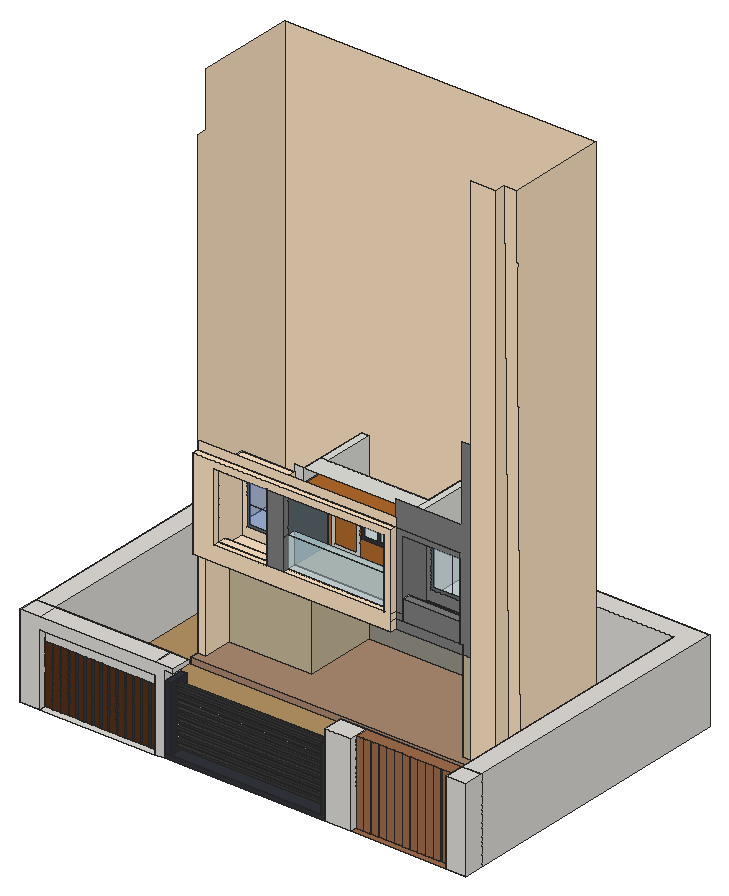
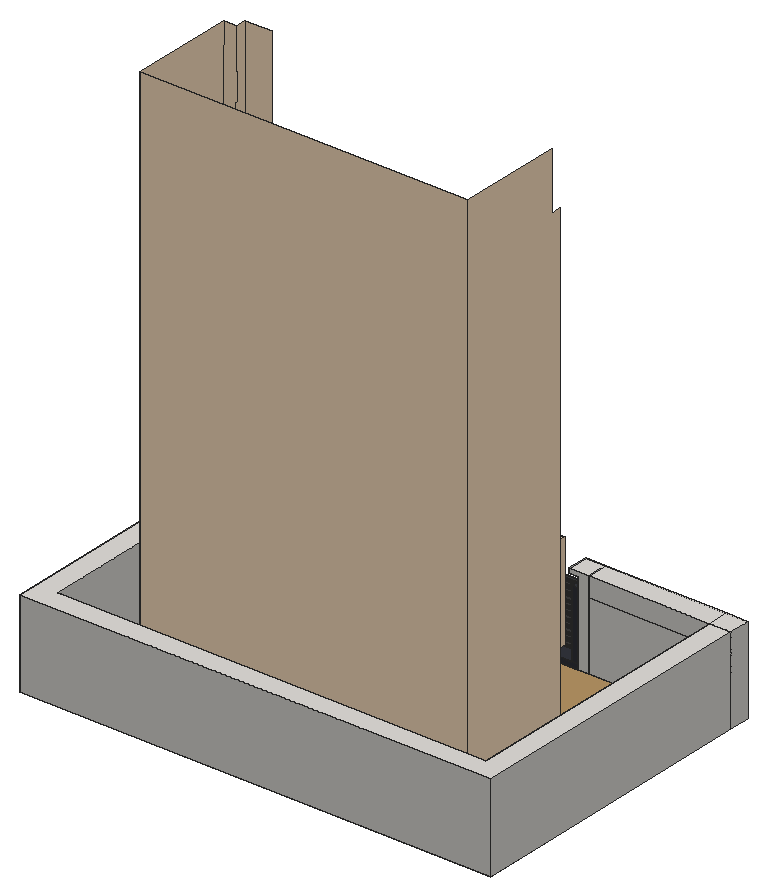
# SketchUp Ruby script. Lengths in inches.
U = 1.inch
M = Sketchup.active_model
def pt(a) = Geom::Point3d.new(a.map { |v| v * U })
def face(e, loops, mat)
  f = e.add_face(loops[0].map { |a| pt(a) })
  loops[1..].each { |l| e.add_face(l.map { |a| pt(a) }).erase! }
  f.material = f.back_material = mat if mat
  f
end
# faces: each face lists its corners as indices into pts; further lists are holes
def faces(e, pts, list, mat = nil) = list.each { |f| face(e, (f[0].is_a?(Array) ? f : [f]).map { |l| l.map { |i| pts[i] } }, mat) }
# xy, xz, yz: faces in a plane at the given z, y or x. An outline is a flat list of corners, or four numbers for a rectangle; further outlines are holes
def ring(l) = l.size == 4 ? [[l[0], l[1]], [l[2], l[1]], [l[2], l[3]], [l[0], l[3]]] : l.each_slice(2).to_a
def flat(e, list, mat, &to3) = list.each { |f| face(e, (f[0].is_a?(Array) ? f : [f]).map { |l| ring(l).map { |u, v| to3.(u, v) } }, mat) }
def xy(e, z, list, mat = nil) = flat(e, list, mat) { |x, y| [x, y, z] }
def xz(e, y, list, mat = nil) = flat(e, list, mat) { |x, z| [x, y, z] }
def yz(e, x, list, mat = nil) = flat(e, list, mat) { |y, z| [x, y, z] }
def lines(e, pts, list) = list.each { |a, b| e.add_line(pt(pts[a]), pt(pts[b])) }
# prism: a flat outline (further loops are holes) pulled along v
def prism(e, loops, v, mat = nil)
  f = face(e, loops, mat); d = Geom::Vector3d.new(v.map { |x| x * U })
  f.pushpull(f.normal.samedirection?(d) ? d.length : -d.length)
end
def box(e, o, s, mat = nil) = prism(e, [[o, [o[0] + s[0], o[1], o[2]], [o[0] + s[0], o[1] + s[1], o[2]], [o[0], o[1] + s[1], o[2]]]], [0, 0, s[2]], mat)
def at(x, y, z, deg = 0) = Geom::Transformation.translation(pt([x, y, z])) * Geom::Transformation.rotation(ORIGIN, Z_AXIS, deg.degrees)
def axes(o, x, y, z) = Geom::Transformation.new([*x, 0, *y, 0, *z, 0, *pt(o).to_a, 1])
def part(name) = M.definitions.add(name)
# library, detail: a bought-in or finely detailed component or shape, given as its bounding box
def library(name, o, s) = part(name).tap { |d| box(d.entities, o, s) }
def detail(e, o, s) = box(e.add_group.entities, o, s)
def put(e, d, t, mat = nil) = e.add_instance(d, t).tap { |i| i.material = mat if mat }
def group(e, t, mat = nil) = e.add_group.tap { |g| g.transformation = t; g.material = mat if mat }.entities
root = M.entities
M.materials.add("[0012_Bisque]").color = [255, 228, 196]
M.materials.add("[Carpet Pattern Leaf Squares Tan]").color = [181, 154, 125]
M.materials.add("[Color M07]").color = [58, 58, 58]
M.materials.add("[Formica Graystone]").color = [149, 146, 135]
M.materials.add("[Formica Laminate Dark]").color = [50, 53, 60]
M.materials.add("[Formica Speckled Grey]").color = [94, 105, 111]
M.materials.add("[Groundcover Sand Smooth]").color = [182, 148, 101]
M.materials.add("[Quartz Light Brown]").color = [199, 184, 152]
M.materials.add("[Slate Light Tile]").color = [127, 127, 127]
M.materials.add("[Terrazzo Tile Accent]").color = [224, 221, 217]
M.materials.add("[Terrazzo Tile Light]").color = [219, 217, 210]
M.materials.add("[Tile Veriegated Stone]").color = [171, 137, 112]
M.materials.add("[Translucent Glass Blue]").color = [100, 149, 237]
M.materials["[Translucent Glass Blue]"].alpha = 0.5
M.materials.add("[Translucent Glass Safety]").color = [204, 235, 244]
M.materials["[Translucent Glass Safety]"].alpha = 0.5
M.materials.add("[Wood Bamboo]").color = [177, 105, 43]
M.materials.add("[Wood Veneer 01]").color = [84, 49, 25]
M.materials.add("[Wood Veneer 02]").color = [160, 108, 76]
xy(root,0,[[0,0,26.06,26.06],[177.43,0,190.63,26.06],[190.63,0,401.35,26.06],[401.35,0,436.18,26.06],[561.76,0,587.8125,26.06],
  [26.06,8.35,177.43,26.06],[436.18,8.57,561.76,26.06],[0,26.06,0,401.5,587.8125,401.5,587.8125,26.06,561.76,26.06,561.76,375.44,26.06,375.44,26.06,26.06],[88.29,171.61,448.4,325.8],[448.4,171.61,498.52,325.8]])
xy(root,0,[[[26.06,26.06,561.76,375.44],[448.4,171.61,498.52,325.8]]],"[Groundcover Sand Smooth]")
xy(root,0,[[26.06,0,177.43,8.35]],"[Terrazzo Tile Accent]")
xy(root,0,[[436.18,0,561.76,8.57]],"[Wood Veneer 02]")
xy(root,6.0625,[[190.63,0,198.32,26.06],[396.54,0,401.35,26.06]])
xy(root,6.0625,[[198.32,0,396.54,26.06]],"[Formica Laminate Dark]")
xy(root,9,[[88.29,171.61,498.52,171.61,498.52,202.27,482.08,202.27,482.08,181.99,438.01,181.99,438.01,315.42,207.7,315.42,207.7,220.49,98.67,220.49,98.67,181.99,88.29,181.99]],"[Tile Veriegated Stone]")
xy(root,12.03,[[198.32,9.24,396.54,13.93]],"[Color M07]")
xy(root,15.03,[[198.32,9.24,396.54,13.93]],"[Color M07]")
xy(root,19.66,[[198.32,9.24,401.35,13.93]],"[Color M07]")
xy(root,22.66,[[198.32,9.24,401.35,13.93]],"[Color M07]")
xy(root,27.1,[[198.32,9.24,396.54,13.93]],"[Color M07]")
xy(root,30.1,[[198.32,9.24,396.54,13.93]],"[Color M07]")
xy(root,33.97,[[198.32,9.24,396.54,13.93]],"[Color M07]")
xy(root,36.97,[[198.32,9.24,396.54,13.93]],"[Color M07]")
xy(root,41.35,[[198.32,9.24,396.54,13.93]],"[Color M07]")
xy(root,44.35,[[198.32,9.24,396.54,13.93]],"[Color M07]")
xy(root,48.91,[[198.32,9.24,396.54,13.93]],"[Color M07]")
xy(root,51.91,[[198.32,9.24,396.54,13.93]],"[Color M07]")
xy(root,55.78,[[198.32,9.24,396.54,13.93]],"[Color M07]")
xy(root,58.78,[[198.32,9.24,396.54,13.93]],"[Color M07]")
xy(root,62.91,[[198.32,9.24,396.54,13.93]],"[Color M07]")
xy(root,65.91,[[198.32,9.24,396.54,13.93]],"[Color M07]")
xy(root,71.22,[[198.32,9.24,396.54,13.93]],"[Color M07]")
xy(root,74.22,[[198.32,9.24,396.54,13.93]],"[Color M07]")
xy(root,78.85,[[198.32,9.24,396.54,13.93]],"[Color M07]")
xy(root,81.85,[[198.32,9.24,396.54,13.93]],"[Color M07]")
xy(root,85.66,[[198.32,9.24,396.54,13.93]],"[Color M07]")
xy(root,88.66,[[198.32,9.24,396.54,13.93]],"[Color M07]")
xy(root,91.76,[[190.63,0,198.32,26.06],[396.54,0,401.35,26.06]],"[Formica Laminate Dark]")
xy(root,93.4375,[[26.06,0,177.43,8.35]])
xy(root,104.12,[[190.63,0,201.76,26.06]])
xy(root,109.3125,[[0,0,26.06,26.06],[26.06,0,177.43,26.06],[177.43,0,201.76,26.06],[401.35,0,436.18,26.06],[561.76,0,587.8125,26.06],
  [0,26.06,26.06,26.06,26.06,375.44,561.76,375.44,561.76,26.06,587.8125,26.06,587.8125,401.5,0,401.5]],"[Terrazzo Tile Accent]")
xy(root,109.3125,[[436.18,8.57,561.76,26.06]],"[Wood Veneer 02]")
xy(root,129,[[88.29,174.18,98.67,181.99],[98.67,174.18,207.7,181.99],[98.67,181.99,207.7,220.49],[98.67,220.49,207.7,315.42]])
xy(root,129,[[207.7,174.18,349.51,181.99],[207.7,181.99,438.01,315.42]],"[0012_Bisque]")
xy(root,141,[[358.38,181.99,434.83,192.87],[434.83,181.99,438.01,192.87],[98.67,192.87,116.04,220.49],[349.51,192.87,358.38,220.49],[434.83,192.87,438.01,220.49],
  [98.67,220.49,197.7,315.42],[349.51,220.49,438.01,315.42],[207.7,247.93,340.25,315.42]])
xy(root,141,[[116.04,192.87,186.07,220.49]],"[0012_Bisque]")
xy(root,149.5,[[186.07,174.18,207.7,181.99],[340.25,174.18,349.51,181.99],[207.7,181.99,340.25,192.87]])
xy(root,149.5,[[116.04,174.18,186.07,181.99],[207.7,174.18,340.25,181.99],[116.04,181.99,186.07,192.87]],"[0012_Bisque]")
xy(root,149.5,[[207.7,192.87,340.25,247.93]],"[Carpet Pattern Leaf Squares Tan]")
xy(root,149.5,[[358.38,192.87,434.83,220.49]],"[Formica Speckled Grey]")
xy(root,167,[[358.38,181.99,434.83,192.87]],"[Slate Light Tile]")
xy(root,189.8125,[[207.7,181.99,340.25,192.87]],"[Translucent Glass Safety]")
xy(root,239.83,[[220.34,200.24,219.16,200.39,218.06,200.85,217.11,201.58,216.39,202.52,215.93,203.62,215.78,204.8,215.93,205.98,216.39,207.08,217.11,208.03,218.06,208.75,219.16,209.21,220.34,209.36,221.52,209.21,222.62,208.75,223.57,208.03,224.29,207.08,224.75,205.98,224.9,204.8,224.75,203.62,224.29,202.52,223.57,201.58,222.62,200.85,221.52,200.39],[270.09,200.24,268.91,200.39,267.81,200.85,266.86,201.58,266.14,202.52,265.68,203.62,265.53,204.8,265.68,205.98,266.14,207.08,266.86,208.03,267.81,208.75,268.91,209.21,270.09,209.36,271.27,209.21,272.37,208.75,273.32,208.03,274.04,207.08,274.5,205.98,274.65,204.8,274.5,203.62,274.04,202.52,273.32,201.58,272.37,200.85,271.27,200.39],[318.46,200.24,317.28,200.39,316.18,200.85,315.24,201.58,314.51,202.52,314.06,203.62,313.9,204.8,314.06,205.98,314.51,207.08,315.24,208.03,316.18,208.75,317.28,209.21,318.46,209.36,319.65,209.21,320.75,208.75,321.69,208.03,322.42,207.08,322.87,205.98,323.03,204.8,322.87,203.62,322.42,202.52,321.69,201.58,320.75,200.85,319.65,200.39]])
xy(root,239.83,[[116.04,174.18,186.07,181.99],[207.7,174.18,340.25,181.99],[116.04,181.99,186.07,220.49]],"[0012_Bisque]")
xy(root,239.83,[[[207.7,181.99,340.25,247.93],[270.09,200.24,271.27,200.39,272.37,200.85,273.32,201.58,274.04,202.52,274.5,203.62,274.65,204.8,274.5,205.98,274.04,207.08,273.32,208.03,272.37,208.75,271.27,209.21,270.09,209.36,268.91,209.21,267.81,208.75,266.86,208.03,266.14,207.08,265.68,205.98,265.53,204.8,265.68,203.62,266.14,202.52,266.86,201.58,267.81,200.85,268.91,200.39],[318.46,200.24,319.65,200.39,320.75,200.85,321.69,201.58,322.42,202.52,322.87,203.62,323.03,204.8,322.87,205.98,322.42,207.08,321.69,208.03,320.75,208.75,319.65,209.21,318.46,209.36,317.28,209.21,316.18,208.75,315.24,208.03,314.51,207.08,314.06,205.98,313.9,204.8,314.06,203.62,314.51,202.52,315.24,201.58,316.18,200.85,317.28,200.39],[220.34,200.24,221.52,200.39,222.62,200.85,223.57,201.58,224.29,202.52,224.75,203.62,224.9,204.8,224.75,205.98,224.29,207.08,223.57,208.03,222.62,208.75,221.52,209.21,220.34,209.36,219.16,209.21,218.06,208.75,217.11,208.03,216.39,207.08,215.93,205.98,215.78,204.8,215.93,203.62,216.39,202.52,217.11,201.58,218.06,200.85,219.16,200.39]]],"[Wood Bamboo]")
xy(root,241.79,[[358.38,181.99,434.83,220.49]],"[Slate Light Tile]")
xy(root,249,[[349.51,181.99,434.83,220.49],[197.7,220.49,340.25,247.93],[340.25,220.49,349.51,315.42],[197.7,247.93,207.7,315.42]])
xy(root,249,[[88.29,174.18,349.51,181.99]],"[0012_Bisque]")
xz(root,0,[[190.63,0,401.35,6.0625],[190.63,6.0625,198.32,91.76],[396.54,6.0625,401.35,91.76]],"[Formica Laminate Dark]")
xz(root,0,[[0,0,26.06,0,26.06,93.4375,177.43,93.4375,177.43,0,190.63,0,190.63,104.12,201.76,104.12,201.76,109.3125,0,109.3125],[401.35,0,436.18,109.3125],[561.76,0,587.8125,109.3125]],"[Terrazzo Tile Accent]")
xz(root,8.35,[[34.49,0,36.74,77.3125],[45.18,0,47.43,77.3125],[55.87,0,58.12,77.3125],[66.56,0,68.81,77.3125],[77.24,0,79.49,77.3125],
  [87.93,0,90.18,77.3125],[98.62,0,100.87,77.3125],[109.31,0,111.56,77.3125],[119.99,0,122.24,77.3125],[130.68,0,132.93,77.3125],
  [141.37,0,143.37,77.3125],[151.81,0,154.12,77.3125],[162.56,0,165.37,77.3125],[173.81,0,177.43,77.3125]],"[Formica Laminate Dark]")
xz(root,8.35,[[26.06,77.3125,177.43,93.4375]],"[Terrazzo Tile Accent]")
xz(root,8.35,[[26.06,0,34.49,77.3125],[36.74,0,45.18,77.3125],[47.43,0,55.87,77.3125],[58.12,0,66.56,77.3125],[68.81,0,77.24,77.3125],
  [79.49,0,87.93,77.3125],[90.18,0,98.62,77.3125],[100.87,0,109.31,77.3125],[111.56,0,119.99,77.3125],[122.24,0,130.68,77.3125],
  [132.93,0,141.37,77.3125],[143.37,0,151.81,77.3125],[154.12,0,162.56,77.3125],[165.37,0,173.81,77.3125]],"[Wood Veneer 01]")
xz(root,8.57,[[444.65,0,446.43,109.3125],[454.9,0,456.68,109.3125],[465.15,0,466.93,109.3125],[475.4,0,477.18,109.3125],[485.65,0,487.43,109.3125],
  [495.9,0,497.68,109.3125],[506.15,0,507.93,109.3125],[516.4,0,518.18,109.3125],[526.65,0,528.43,109.3125],[536.9,0,538.68,109.3125],
  [547.15,0,550.43,109.3125],[558.9,0,561.76,109.3125]],"[Formica Laminate Dark]")
xz(root,8.57,[[436.18,0,444.65,109.3125],[446.43,0,454.9,109.3125],[456.68,0,465.15,109.3125],[466.93,0,475.4,109.3125],[477.18,0,485.65,109.3125],
  [487.43,0,495.9,109.3125],[497.68,0,506.15,109.3125],[507.93,0,516.4,109.3125],[518.18,0,526.65,109.3125],[528.43,0,536.9,109.3125],
  [538.68,0,547.15,109.3125],[550.43,0,558.9,109.3125]],"[Wood Veneer 02]")
xz(root,9.24,[[198.32,12.03,396.54,15.03],[198.32,19.66,401.35,22.66],[198.32,27.1,396.54,30.1],[198.32,33.97,396.54,36.97],[198.32,41.35,396.54,44.35],
  [198.32,48.91,396.54,51.91],[198.32,55.78,396.54,58.78],[198.32,62.91,396.54,65.91],[198.32,71.22,396.54,74.22],[198.32,78.85,396.54,81.85],
  [198.32,85.66,396.54,88.66]],"[Color M07]")
xz(root,13.93,[[198.32,12.03,396.54,15.03],[198.32,19.66,401.35,22.66],[198.32,27.1,396.54,30.1],[198.32,33.97,396.54,36.97],[198.32,41.35,396.54,44.35],
  [198.32,48.91,396.54,51.91],[198.32,55.78,396.54,58.78],[198.32,62.91,396.54,65.91],[198.32,71.22,396.54,74.22],[198.32,78.85,396.54,81.85],
  [198.32,85.66,396.54,88.66]],"[Color M07]")
xz(root,26.06,[[0,0,26.06,109.3125],[561.76,0,587.8125,109.3125]])
xz(root,26.06,[[190.63,0,401.35,6.0625],[190.63,6.0625,198.32,91.76],[396.54,6.0625,401.35,91.76]],"[Formica Laminate Dark]")
xz(root,26.06,[[26.06,0,177.43,84.72],[177.43,0,177.43,109.3125,201.76,109.3125,201.76,104.12,190.63,104.12,190.63,0],[401.35,0,436.18,109.3125],[436.18,0,561.76,109.3125],[26.06,84.72,177.43,109.3125]],"[Terrazzo Tile Accent]")
xz(root,171.61,[[88.29,0,498.52,9]],"[Tile Veriegated Stone]")
xz(root,174.18,[[88.29,129,349.51,129,349.51,149.5,116.04,149.5,116.04,239.83,340.25,239.83,340.25,149.5,349.51,149.5,349.51,249,88.29,249]],"[0012_Bisque]")
xz(root,174.18,[[186.07,149.5,207.7,239.83]],"[Slate Light Tile]")
xz(root,181.99,[[88.29,129,88.29,249,349.51,249,349.51,149.5,340.25,149.5,340.25,239.83,207.7,239.83,207.7,149.5,186.07,149.5,186.07,239.83,116.04,239.83,116.04,149.5,349.51,149.5,349.51,129]])
xz(root,181.99,[[88.29,9,98.67,129],[448.4,9,482.08,693],[88.29,249,349.51,261]],"[0012_Bisque]")
xz(root,181.99,[[438.01,9,448.4,129]],"[Quartz Light Brown]")
xz(root,181.99,[[349.51,129,438.01,141],[438.01,129,448.4,129,448.4,381,437.4,381,437.4,282.375,349.51,282.375,349.51,249,434.83,249,434.83,141,438.01,141],[349.51,141,358.38,149.5],[358.38,141,434.83,167],[349.51,149.5,358.38,149.5,358.38,241.79,434.83,241.79,434.83,249,349.51,249]],"[Slate Light Tile]")
xz(root,181.99,[[207.7,149.5,340.25,189.8125]],"[Translucent Glass Safety]")
xz(root,192.87,[[116.04,141,186.07,149.5],[358.38,141,434.83,149.5],[358.38,149.5,434.83,167]])
xz(root,192.87,[[207.7,149.5,340.25,189.8125]],"[Translucent Glass Safety]")
xz(root,220.49,[[186.07,141,197.7,249],[349.51,141,358.38,141,358.38,241.79,434.83,241.79,434.83,249,349.51,249],[358.38,141,434.83,149.5]])
xz(root,220.49,[[[116.04,141,186.07,239.83],[122.5,152.41,178.75,228.41]]],"[0012_Bisque]")
xz(root,220.49,[[[122.5,152.41,178.75,228.41],[126.28,156.19,174.97,224.63]],[[365.65,164.13,422.77,230.07],[369.44,167.93,418.98,226.28]]],"[Formica Speckled Grey]")
xz(root,220.49,[[98.67,9,207.7,129]],"[Quartz Light Brown]")
xz(root,220.49,[[[358.38,149.5,434.83,241.79],[365.65,164.13,422.77,230.07]]],"[Slate Light Tile]")
xz(root,220.49,[[126.28,156.19,150.625,180.17],[150.625,156.19,174.97,180.17],[126.28,180.17,150.625,224.63],[150.625,180.17,174.97,224.63]],"[Translucent Glass Blue]")
xz(root,220.49,[[369.44,167.93,394.21,226.28],[394.21,167.93,418.98,226.28]],"[Translucent Glass Safety]")
xz(root,247.93,[[207.7,141,340.25,149.5],[207.7,239.83,340.25,249]])
xz(root,247.93,[[[252.75,172.43,335.9375,230.62],[256.24,175.92,332.45,227.125]],[273.92,175.92,276.74,227.125],[294.35,175.92,297.33,227.125],[312.07,175.92,314.89,227.125]],"[Formica Laminate Dark]")
xz(root,247.93,[[[212.16,149.5,249.97,235.6875],[216.47,153.81,245.67,231.38]]],"[Terrazzo Tile Light]")
xz(root,247.93,[[256.24,175.92,273.92,227.125],[276.74,175.92,294.35,227.125],[297.33,175.92,312.07,227.125],[314.89,175.92,332.45,227.125]],"[Translucent Glass Safety]")
xz(root,247.93,[[[207.7,149.5,212.16,149.5,212.16,235.6875,249.97,235.6875,249.97,149.5,340.25,149.5,340.25,239.83,207.7,239.83],[252.75,172.43,335.9375,230.62]],[216.47,153.81,245.67,231.38]],"[Wood Bamboo]")
xz(root,315.42,[[98.67,129,98.67,141,197.7,141,197.7,249,207.7,249,207.7,129],[207.7,129,340.25,141],[340.25,129,349.51,249],[349.51,129,438.01,141]])
xz(root,315.42,[[207.7,9,438.01,129]],"[Formica Graystone]")
xz(root,325.8,[[88.29,0,498.52,693]],"[0012_Bisque]")
xz(root,375.44,[[26.06,0,561.76,109.3125]],"[Terrazzo Tile Accent]")
xz(root,401.5,[[0,0,587.8125,109.3125]],"[Terrazzo Tile Accent]")
yz(root,0,[[0,0,26.06,109.3125],[26.06,0,401.5,109.3125]],"[Terrazzo Tile Accent]")
yz(root,26.06,[[8.35,0,26.06,84.72]])
yz(root,26.06,[[0,0,8.35,93.4375],[26.06,0,375.44,109.3125]],"[Terrazzo Tile Accent]")
yz(root,88.29,[[171.61,0,171.61,9,181.99,9,181.99,621,195.54,621,195.54,693,325.8,693,325.8,0],[174.18,129,181.99,249]],"[0012_Bisque]")
yz(root,98.67,[[220.49,129,315.42,141]])
yz(root,98.67,[[181.99,9,220.49,129]],"[0012_Bisque]")
yz(root,116.04,[[192.87,141,220.49,141,220.49,239.83,181.99,239.83,181.99,149.5,192.87,149.5],[174.18,149.5,181.99,239.83]],"[0012_Bisque]")
yz(root,177.43,[[8.35,0,26.06,84.72],[8.35,84.72,26.06,109.3125]])
yz(root,177.43,[[0,0,8.35,93.4375]],"[Terrazzo Tile Accent]")
yz(root,186.07,[[192.87,141,192.87,149.5,181.99,149.5,181.99,239.83,220.49,239.83,220.49,141]],"[0012_Bisque]")
yz(root,186.07,[[174.18,149.5,181.99,239.83]],"[Slate Light Tile]")
yz(root,190.63,[[0,0,26.06,6.0625],[0,6.0625,26.06,91.76]])
yz(root,190.63,[[0,91.76,26.06,104.12]],"[Terrazzo Tile Accent]")
yz(root,197.7,[[220.49,141,315.42,249]])
yz(root,198.32,[[9.24,12.03,13.93,15.03],[9.24,19.66,13.93,22.66],[9.24,27.1,13.93,30.1],[9.24,33.97,13.93,36.97],[9.24,41.35,13.93,44.35],
  [9.24,48.91,13.93,51.91],[9.24,55.78,13.93,58.78],[9.24,62.91,13.93,65.91],[9.24,71.22,13.93,74.22],[9.24,78.85,13.93,81.85],
  [9.24,85.66,13.93,88.66]])
yz(root,198.32,[[[0,6.0625,26.06,91.76],[9.24,85.66,13.93,88.66],[9.24,12.03,13.93,15.03],[9.24,78.85,13.93,81.85],[9.24,19.66,13.93,22.66],[9.24,71.22,13.93,74.22],[9.24,27.1,13.93,30.1],[9.24,62.91,13.93,65.91],[9.24,33.97,13.93,36.97],[9.24,55.78,13.93,58.78],[9.24,41.35,13.93,44.35],[9.24,48.91,13.93,51.91]]],"[Formica Laminate Dark]")
yz(root,201.76,[[0,104.12,26.06,109.3125]],"[Terrazzo Tile Accent]")
yz(root,207.7,[[247.93,141,315.42,249],[181.99,149.5,192.87,189.8125]])
yz(root,207.7,[[192.87,149.5,247.93,149.5,247.93,239.83,181.99,239.83,181.99,189.8125,192.87,189.8125]],"[Formica Speckled Grey]")
yz(root,207.7,[[220.49,9,315.42,129]],"[Quartz Light Brown]")
yz(root,207.7,[[174.18,149.5,181.99,189.8125],[174.18,189.8125,181.99,239.83]],"[Slate Light Tile]")
yz(root,340.25,[[247.93,141,315.42,249],[174.18,149.5,181.99,189.8125],[181.99,149.5,192.87,189.8125]])
yz(root,340.25,[[174.18,189.8125,181.99,239.83]],"[0012_Bisque]")
yz(root,340.25,[[192.87,149.5,192.87,189.8125,181.99,189.8125,181.99,239.83,247.93,239.83,247.93,149.5]],"[Wood Bamboo]")
yz(root,349.51,[[220.49,141,315.42,249]])
yz(root,349.51,[[174.18,129,181.99,141],[174.18,141,181.99,149.5],[174.18,149.5,181.99,249]],"[0012_Bisque]")
yz(root,358.38,[[181.99,141,192.87,167],[192.87,141,220.49,149.5]])
yz(root,358.38,[[192.87,149.5,220.49,149.5,220.49,241.79,181.99,241.79,181.99,167,192.87,167]],"[Slate Light Tile]")
yz(root,396.54,[[[0,6.0625,26.06,91.76],[9.24,85.66,13.93,88.66],[9.24,78.85,13.93,81.85],[9.24,71.22,13.93,74.22],[9.24,62.91,13.93,65.91],[9.24,55.78,13.93,58.78],[9.24,48.91,13.93,51.91],[9.24,41.35,13.93,44.35],[9.24,33.97,13.93,36.97],[9.24,27.1,13.93,30.1],[9.24,12.03,13.93,15.03]]],"[Formica Laminate Dark]")
yz(root,401.35,[[0,0,26.06,6.0625],[[0,6.0625,26.06,91.76],[9.24,19.66,13.93,22.66]]])
yz(root,401.35,[[0,91.76,26.06,109.3125]],"[Terrazzo Tile Accent]")
yz(root,434.83,[[181.99,141,192.87,167],[192.87,141,220.49,149.5]])
yz(root,434.83,[[192.87,149.5,192.87,167,181.99,167,181.99,241.79,220.49,241.79,220.49,149.5]],"[Slate Light Tile]")
yz(root,436.18,[[8.57,0,26.06,109.3125]])
yz(root,436.18,[[0,0,8.57,109.3125]],"[Terrazzo Tile Accent]")
yz(root,438.01,[[181.99,129,220.49,141],[220.49,129,315.42,141]])
yz(root,438.01,[[181.99,9,315.42,129]],"[Formica Graystone]")
yz(root,482.08,[[181.99,9,202.27,9,195.54,693,181.99,693]],"[0012_Bisque]")
yz(root,498.52,[[171.61,0,202.36,0,202.27,9,171.61,9]])
yz(root,498.52,[[202.36,0,325.8,0,325.8,693,195.54,693,202.27,9]],"[0012_Bisque]")
yz(root,561.76,[[8.57,0,26.06,109.3125]])
yz(root,561.76,[[0,0,8.57,109.3125],[26.06,0,375.44,109.3125]],"[Terrazzo Tile Accent]")
yz(root,587.8125,[[0,0,26.06,109.3125],[26.06,0,401.5,109.3125]],"[Terrazzo Tile Accent]")
p = [[482.08,202.27,9],[498.52,202.27,9],[498.52,195.54,693],[482.08,195.54,693],[98.67,181.99,141],[98.67,192.87,141],
  [116.04,181.99,141],[116.04,192.87,141],[349.51,192.87,141],[349.51,181.99,141]]
faces(root,p,[[0,1,2,3]],"[0012_Bisque]")
lines(root,p,[[4,5],[6,7],[8,9]])
